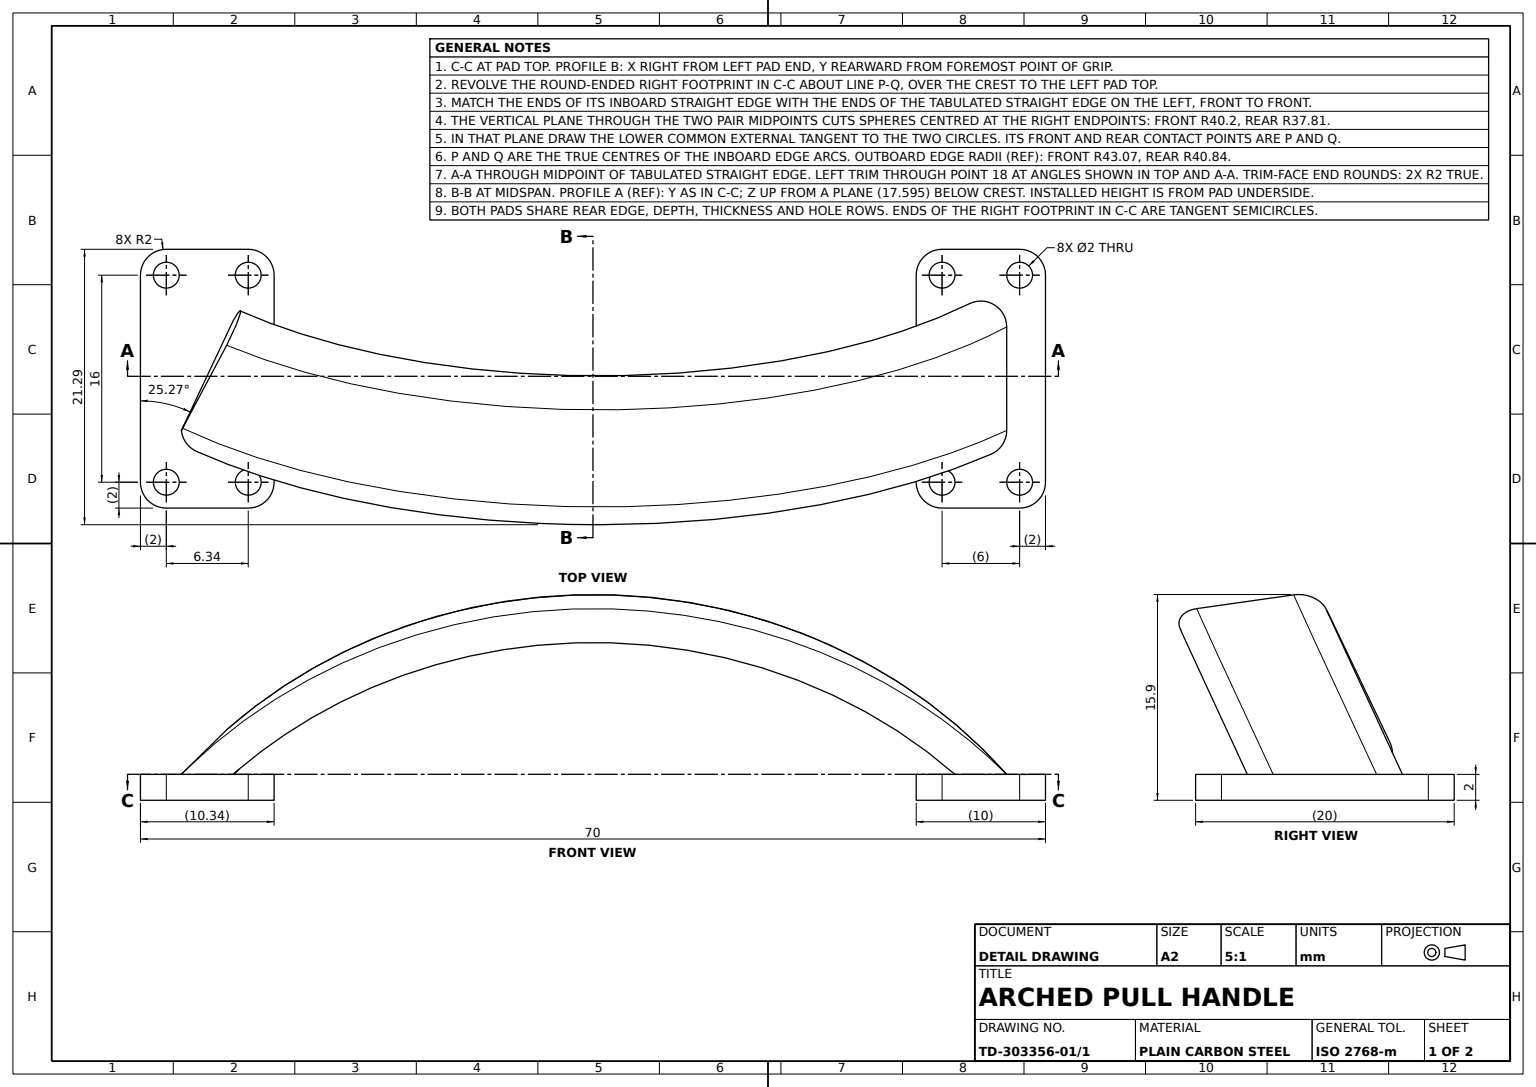
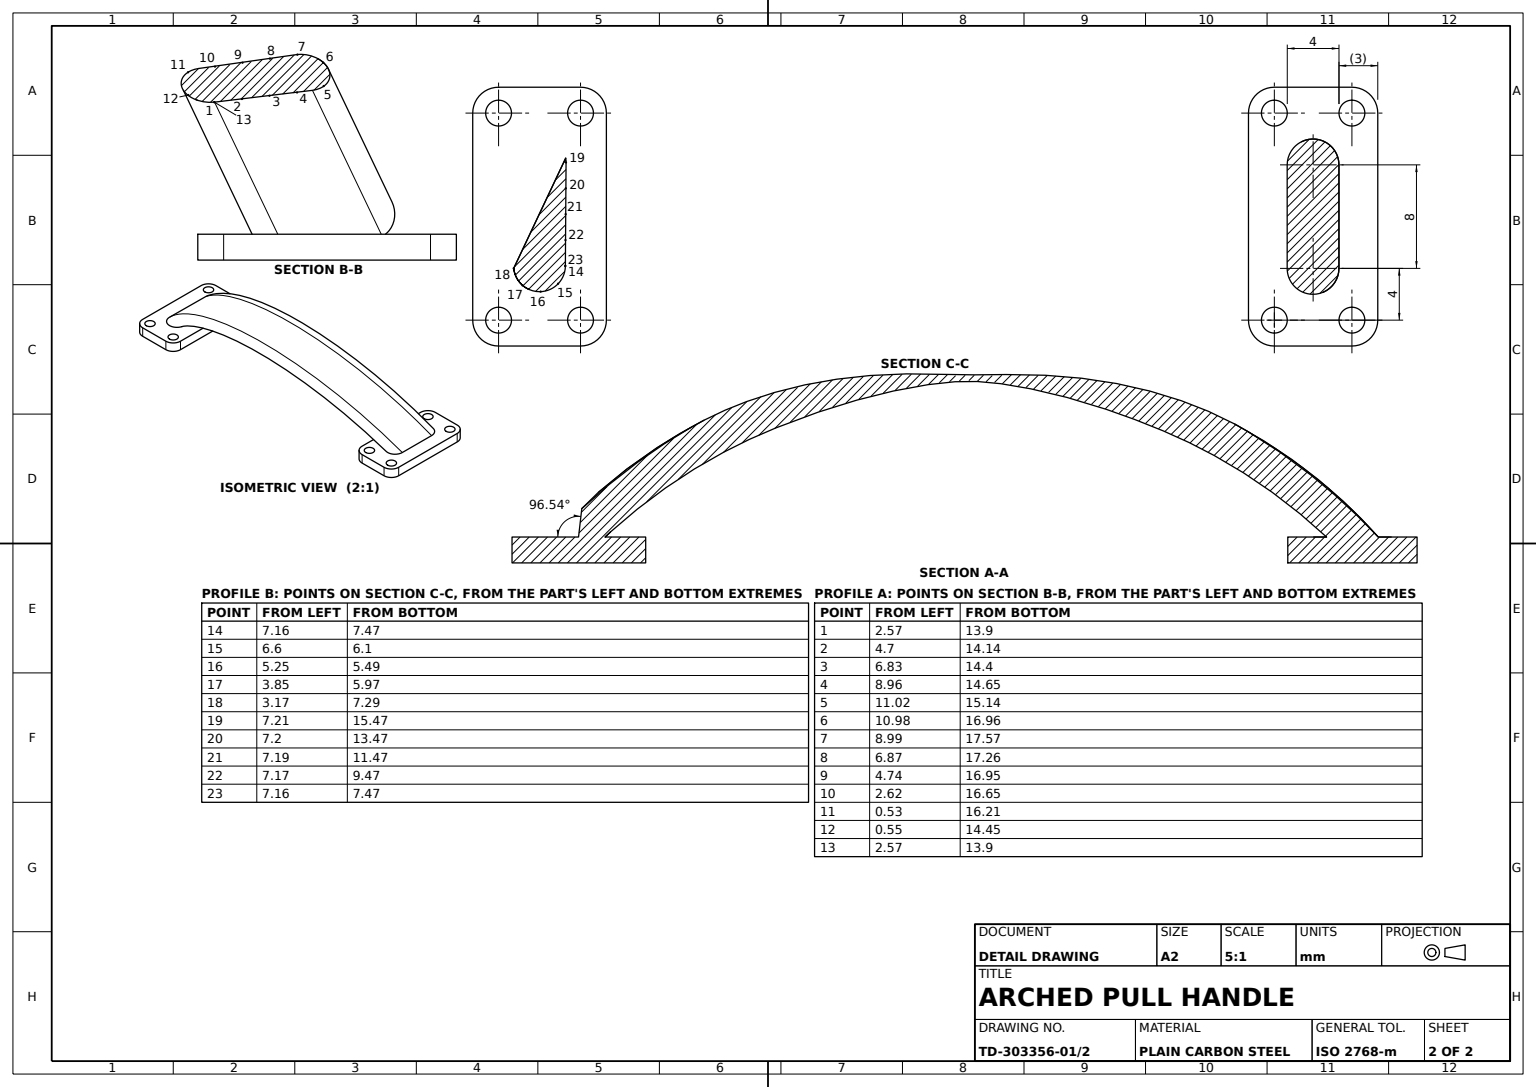
ISO-10303-21;
HEADER;
FILE_DESCRIPTION((''),'2;1');
FILE_NAME('','',(''),(''),'','','');
FILE_SCHEMA(('AUTOMOTIVE_DESIGN'));
ENDSEC;
DATA;
#1=APPLICATION_CONTEXT('');
#2=PRODUCT_CONTEXT('',#1,'mechanical');
#3=PRODUCT('','','',(#2));
#4=PRODUCT_DEFINITION_FORMATION('','',#3);
#5=PRODUCT_DEFINITION_CONTEXT('',#1,'design');
#6=PRODUCT_DEFINITION('','',#4,#5);
#7=PRODUCT_DEFINITION_SHAPE('','',#6);
#8=(LENGTH_UNIT()NAMED_UNIT(*)SI_UNIT(.MILLI.,.METRE.));
#9=(NAMED_UNIT(*)PLANE_ANGLE_UNIT()SI_UNIT($,.RADIAN.));
#10=(NAMED_UNIT(*)SI_UNIT($,.STERADIAN.)SOLID_ANGLE_UNIT());
#11=UNCERTAINTY_MEASURE_WITH_UNIT(LENGTH_MEASURE(1.E-05),#8,'distance_accuracy_value','');
#12=(GEOMETRIC_REPRESENTATION_CONTEXT(3)GLOBAL_UNCERTAINTY_ASSIGNED_CONTEXT((#11))GLOBAL_UNIT_ASSIGNED_CONTEXT((#8,#9,#10))REPRESENTATION_CONTEXT('',''));
#13=CARTESIAN_POINT('',(61.598057,2.,-9.));
#14=VERTEX_POINT('',#13);
#15=CARTESIAN_POINT('',(61.598057,0.,-9.));
#16=VERTEX_POINT('',#15);
#17=CARTESIAN_POINT('',(61.598057,6.,-9.));
#18=DIRECTION('',(0.,-1.,0.));
#19=VECTOR('',#18,1000.);
#20=LINE('',#17,#19);
#21=EDGE_CURVE('',#14,#16,#20,.T.);
#22=ORIENTED_EDGE('',*,*,#21,.T.);
#23=CARTESIAN_POINT('',(61.598057,0.,-7.));
#24=VERTEX_POINT('',#23);
#25=CARTESIAN_POINT('',(61.598057,0.,-8.));
#26=DIRECTION('',(0.,0.,1.));
#27=AXIS2_PLACEMENT_3D('',#25,#18,#26);
#28=CIRCLE('',#27,1.);
#29=EDGE_CURVE('',#16,#24,#28,.T.);
#30=ORIENTED_EDGE('',*,*,#29,.T.);
#31=CARTESIAN_POINT('',(61.598057,2.,-7.));
#32=VERTEX_POINT('',#31);
#33=CARTESIAN_POINT('',(61.598057,6.,-7.));
#34=LINE('',#33,#19);
#35=EDGE_CURVE('',#32,#24,#34,.T.);
#36=ORIENTED_EDGE('',*,*,#35,.F.);
#37=CARTESIAN_POINT('',(61.598057,2.,-8.));
#38=AXIS2_PLACEMENT_3D('',#37,#18,#26);
#39=CIRCLE('',#38,1.);
#40=EDGE_CURVE('',#14,#32,#39,.T.);
#41=ORIENTED_EDGE('',*,*,#40,.F.);
#42=EDGE_LOOP('',(#22,#30,#36,#41));
#43=FACE_OUTER_BOUND('',#42,.T.);
#44=CARTESIAN_POINT('',(61.598057,6.,-8.));
#45=DIRECTION('',(0.,0.,-1.));
#46=AXIS2_PLACEMENT_3D('',#44,#18,#45);
#47=CYLINDRICAL_SURFACE('',#46,1.);
#48=ADVANCED_FACE('',(#43),#47,.F.);
#49=CARTESIAN_POINT('',(61.598057,0.,10.));
#50=VERTEX_POINT('',#49);
#51=CARTESIAN_POINT('',(55.598057,0.,10.));
#52=VERTEX_POINT('',#51);
#53=CARTESIAN_POINT('',(0.,0.,10.));
#54=DIRECTION('',(-1.,0.,0.));
#55=VECTOR('',#54,1000.);
#56=LINE('',#53,#55);
#57=EDGE_CURVE('',#50,#52,#56,.T.);
#58=ORIENTED_EDGE('',*,*,#57,.F.);
#59=CARTESIAN_POINT('',(61.598057,2.,10.));
#60=VERTEX_POINT('',#59);
#61=DIRECTION('',(0.,1.,0.));
#62=VECTOR('',#61,1000.);
#63=LINE('',#49,#62);
#64=EDGE_CURVE('',#50,#60,#63,.T.);
#65=ORIENTED_EDGE('',*,*,#64,.T.);
#66=CARTESIAN_POINT('',(55.598057,2.,10.));
#67=VERTEX_POINT('',#66);
#68=CARTESIAN_POINT('',(0.,2.,10.));
#69=LINE('',#68,#55);
#70=EDGE_CURVE('',#60,#67,#69,.T.);
#71=ORIENTED_EDGE('',*,*,#70,.T.);
#72=LINE('',#51,#62);
#73=EDGE_CURVE('',#52,#67,#72,.T.);
#74=ORIENTED_EDGE('',*,*,#73,.F.);
#75=EDGE_LOOP('',(#58,#65,#71,#74));
#76=FACE_OUTER_BOUND('',#75,.T.);
#77=AXIS2_PLACEMENT_3D('',#53,#45,#54);
#78=PLANE('',#77);
#79=ADVANCED_FACE('',(#76),#78,.F.);
#80=CARTESIAN_POINT('',(1.935999,2.,-7.));
#81=VERTEX_POINT('',#80);
#82=CARTESIAN_POINT('',(1.935999,0.,-7.));
#83=VERTEX_POINT('',#82);
#84=CARTESIAN_POINT('',(1.935999,23.,-7.));
#85=LINE('',#84,#19);
#86=EDGE_CURVE('',#81,#83,#85,.T.);
#87=ORIENTED_EDGE('',*,*,#86,.T.);
#88=CARTESIAN_POINT('',(1.935999,0.,-9.));
#89=VERTEX_POINT('',#88);
#90=CARTESIAN_POINT('',(1.935999,0.,-8.));
#91=AXIS2_PLACEMENT_3D('',#90,#18,#26);
#92=CIRCLE('',#91,1.);
#93=EDGE_CURVE('',#83,#89,#92,.T.);
#94=ORIENTED_EDGE('',*,*,#93,.T.);
#95=CARTESIAN_POINT('',(1.935999,2.,-9.));
#96=VERTEX_POINT('',#95);
#97=CARTESIAN_POINT('',(1.935999,23.,-9.));
#98=LINE('',#97,#19);
#99=EDGE_CURVE('',#96,#89,#98,.T.);
#100=ORIENTED_EDGE('',*,*,#99,.F.);
#101=CARTESIAN_POINT('',(1.935999,2.,-8.));
#102=AXIS2_PLACEMENT_3D('',#101,#18,#26);
#103=CIRCLE('',#102,1.);
#104=EDGE_CURVE('',#81,#96,#103,.T.);
#105=ORIENTED_EDGE('',*,*,#104,.F.);
#106=EDGE_LOOP('',(#87,#94,#100,#105));
#107=FACE_OUTER_BOUND('',#106,.T.);
#108=CARTESIAN_POINT('',(1.935999,23.,-8.));
#109=AXIS2_PLACEMENT_3D('',#108,#18,#45);
#110=CYLINDRICAL_SURFACE('',#109,1.);
#111=ADVANCED_FACE('',(#107),#110,.F.);
#112=CARTESIAN_POINT('',(61.598057,0.,7.));
#113=VERTEX_POINT('',#112);
#114=CARTESIAN_POINT('',(61.598057,0.,9.));
#115=VERTEX_POINT('',#114);
#116=CARTESIAN_POINT('',(61.598057,0.,8.));
#117=AXIS2_PLACEMENT_3D('',#116,#18,#26);
#118=CIRCLE('',#117,1.);
#119=EDGE_CURVE('',#113,#115,#118,.T.);
#120=ORIENTED_EDGE('',*,*,#119,.F.);
#121=EDGE_CURVE('',#115,#113,#118,.T.);
#122=ORIENTED_EDGE('',*,*,#121,.F.);
#123=EDGE_LOOP('',(#120,#122));
#124=FACE_BOUND('',#123,.T.);
#125=CARTESIAN_POINT('',(55.598057,0.,-9.));
#126=VERTEX_POINT('',#125);
#127=CARTESIAN_POINT('',(55.598057,0.,-7.));
#128=VERTEX_POINT('',#127);
#129=CARTESIAN_POINT('',(55.598057,0.,-8.));
#130=AXIS2_PLACEMENT_3D('',#129,#18,#26);
#131=CIRCLE('',#130,1.);
#132=EDGE_CURVE('',#126,#128,#131,.T.);
#133=ORIENTED_EDGE('',*,*,#132,.F.);
#134=EDGE_CURVE('',#128,#126,#131,.T.);
#135=ORIENTED_EDGE('',*,*,#134,.F.);
#136=EDGE_LOOP('',(#133,#135));
#137=FACE_BOUND('',#136,.T.);
#138=CARTESIAN_POINT('',(63.598057,0.,8.));
#139=VERTEX_POINT('',#138);
#140=CIRCLE('',#117,2.);
#141=EDGE_CURVE('',#139,#50,#140,.T.);
#142=ORIENTED_EDGE('',*,*,#141,.T.);
#143=ORIENTED_EDGE('',*,*,#57,.T.);
#144=CARTESIAN_POINT('',(53.598057,0.,8.));
#145=VERTEX_POINT('',#144);
#146=CARTESIAN_POINT('',(55.598057,0.,8.));
#147=AXIS2_PLACEMENT_3D('',#146,#18,#26);
#148=CIRCLE('',#147,2.);
#149=EDGE_CURVE('',#52,#145,#148,.T.);
#150=ORIENTED_EDGE('',*,*,#149,.T.);
#151=CARTESIAN_POINT('',(53.598057,0.,-8.));
#152=VERTEX_POINT('',#151);
#153=CARTESIAN_POINT('',(53.598057,0.,0.));
#154=VECTOR('',#26,1000.);
#155=LINE('',#153,#154);
#156=EDGE_CURVE('',#152,#145,#155,.T.);
#157=ORIENTED_EDGE('',*,*,#156,.F.);
#158=CARTESIAN_POINT('',(55.598057,0.,-10.));
#159=VERTEX_POINT('',#158);
#160=AXIS2_PLACEMENT_3D('',#129,#61,#26);
#161=CIRCLE('',#160,2.);
#162=EDGE_CURVE('',#159,#152,#161,.T.);
#163=ORIENTED_EDGE('',*,*,#162,.F.);
#164=CARTESIAN_POINT('',(61.598057,0.,-10.));
#165=VERTEX_POINT('',#164);
#166=CARTESIAN_POINT('',(0.,0.,-10.));
#167=LINE('',#166,#55);
#168=EDGE_CURVE('',#165,#159,#167,.T.);
#169=ORIENTED_EDGE('',*,*,#168,.F.);
#170=CARTESIAN_POINT('',(63.598057,0.,-8.));
#171=VERTEX_POINT('',#170);
#172=CIRCLE('',#27,2.);
#173=EDGE_CURVE('',#165,#171,#172,.T.);
#174=ORIENTED_EDGE('',*,*,#173,.T.);
#175=CARTESIAN_POINT('',(63.598057,0.,0.));
#176=LINE('',#175,#154);
#177=EDGE_CURVE('',#171,#139,#176,.T.);
#178=ORIENTED_EDGE('',*,*,#177,.T.);
#179=EDGE_LOOP('',(#142,#143,#150,#157,#163,#169,#174,#178));
#180=FACE_OUTER_BOUND('',#179,.T.);
#181=EDGE_CURVE('',#24,#16,#28,.T.);
#182=ORIENTED_EDGE('',*,*,#181,.F.);
#183=ORIENTED_EDGE('',*,*,#29,.F.);
#184=EDGE_LOOP('',(#182,#183));
#185=FACE_BOUND('',#184,.T.);
#186=CARTESIAN_POINT('',(55.598057,0.,7.));
#187=VERTEX_POINT('',#186);
#188=CARTESIAN_POINT('',(55.598057,0.,9.));
#189=VERTEX_POINT('',#188);
#190=CIRCLE('',#147,1.);
#191=EDGE_CURVE('',#187,#189,#190,.T.);
#192=ORIENTED_EDGE('',*,*,#191,.F.);
#193=EDGE_CURVE('',#189,#187,#190,.T.);
#194=ORIENTED_EDGE('',*,*,#193,.F.);
#195=EDGE_LOOP('',(#192,#194));
#196=FACE_BOUND('',#195,.T.);
#197=CARTESIAN_POINT('',(0.,0.,0.));
#198=AXIS2_PLACEMENT_3D('',#197,#61,#26);
#199=PLANE('',#198);
#200=ADVANCED_FACE('',(#124,#137,#180,#185,#196),#199,.F.);
#201=CARTESIAN_POINT('',(-4.401943,0.,-10.));
#202=VERTEX_POINT('',#201);
#203=CARTESIAN_POINT('',(-6.401943,0.,-8.));
#204=VERTEX_POINT('',#203);
#205=CARTESIAN_POINT('',(-4.401943,0.,-8.));
#206=AXIS2_PLACEMENT_3D('',#205,#61,#26);
#207=CIRCLE('',#206,2.);
#208=EDGE_CURVE('',#202,#204,#207,.T.);
#209=ORIENTED_EDGE('',*,*,#208,.F.);
#210=CARTESIAN_POINT('',(1.935999,0.,-10.));
#211=VERTEX_POINT('',#210);
#212=LINE('',#201,#55);
#213=EDGE_CURVE('',#211,#202,#212,.T.);
#214=ORIENTED_EDGE('',*,*,#213,.F.);
#215=CARTESIAN_POINT('',(3.935999,0.,-8.));
#216=VERTEX_POINT('',#215);
#217=AXIS2_PLACEMENT_3D('',#90,#61,#26);
#218=CIRCLE('',#217,2.);
#219=EDGE_CURVE('',#216,#211,#218,.T.);
#220=ORIENTED_EDGE('',*,*,#219,.F.);
#221=CARTESIAN_POINT('',(3.935999,0.,8.));
#222=VERTEX_POINT('',#221);
#223=VECTOR('',#45,1000.);
#224=LINE('',#215,#223);
#225=EDGE_CURVE('',#222,#216,#224,.T.);
#226=ORIENTED_EDGE('',*,*,#225,.F.);
#227=CARTESIAN_POINT('',(1.935999,0.,10.));
#228=VERTEX_POINT('',#227);
#229=CARTESIAN_POINT('',(1.935999,0.,8.));
#230=AXIS2_PLACEMENT_3D('',#229,#61,#26);
#231=CIRCLE('',#230,2.);
#232=EDGE_CURVE('',#228,#222,#231,.T.);
#233=ORIENTED_EDGE('',*,*,#232,.F.);
#234=CARTESIAN_POINT('',(-4.401943,0.,10.));
#235=VERTEX_POINT('',#234);
#236=DIRECTION('',(1.,0.,0.));
#237=VECTOR('',#236,1000.);
#238=LINE('',#234,#237);
#239=EDGE_CURVE('',#235,#228,#238,.T.);
#240=ORIENTED_EDGE('',*,*,#239,.F.);
#241=CARTESIAN_POINT('',(-6.401943,0.,8.));
#242=VERTEX_POINT('',#241);
#243=CARTESIAN_POINT('',(-4.401943,0.,8.));
#244=AXIS2_PLACEMENT_3D('',#243,#61,#26);
#245=CIRCLE('',#244,2.);
#246=EDGE_CURVE('',#242,#235,#245,.T.);
#247=ORIENTED_EDGE('',*,*,#246,.F.);
#248=LINE('',#203,#154);
#249=EDGE_CURVE('',#204,#242,#248,.T.);
#250=ORIENTED_EDGE('',*,*,#249,.F.);
#251=EDGE_LOOP('',(#209,#214,#220,#226,#233,#240,#247,#250));
#252=FACE_OUTER_BOUND('',#251,.T.);
#253=CARTESIAN_POINT('',(-4.401943,0.,7.));
#254=VERTEX_POINT('',#253);
#255=CARTESIAN_POINT('',(-4.401943,0.,9.));
#256=VERTEX_POINT('',#255);
#257=AXIS2_PLACEMENT_3D('',#243,#18,#26);
#258=CIRCLE('',#257,1.);
#259=EDGE_CURVE('',#254,#256,#258,.T.);
#260=ORIENTED_EDGE('',*,*,#259,.F.);
#261=EDGE_CURVE('',#256,#254,#258,.T.);
#262=ORIENTED_EDGE('',*,*,#261,.F.);
#263=EDGE_LOOP('',(#260,#262));
#264=FACE_BOUND('',#263,.T.);
#265=CARTESIAN_POINT('',(1.935999,0.,9.));
#266=VERTEX_POINT('',#265);
#267=CARTESIAN_POINT('',(1.935999,0.,7.));
#268=VERTEX_POINT('',#267);
#269=AXIS2_PLACEMENT_3D('',#229,#18,#26);
#270=CIRCLE('',#269,1.);
#271=EDGE_CURVE('',#266,#268,#270,.T.);
#272=ORIENTED_EDGE('',*,*,#271,.F.);
#273=EDGE_CURVE('',#268,#266,#270,.T.);
#274=ORIENTED_EDGE('',*,*,#273,.F.);
#275=EDGE_LOOP('',(#272,#274));
#276=FACE_BOUND('',#275,.T.);
#277=CARTESIAN_POINT('',(-4.401943,0.,-9.));
#278=VERTEX_POINT('',#277);
#279=CARTESIAN_POINT('',(-4.401943,0.,-7.));
#280=VERTEX_POINT('',#279);
#281=AXIS2_PLACEMENT_3D('',#205,#18,#26);
#282=CIRCLE('',#281,1.);
#283=EDGE_CURVE('',#278,#280,#282,.T.);
#284=ORIENTED_EDGE('',*,*,#283,.F.);
#285=EDGE_CURVE('',#280,#278,#282,.T.);
#286=ORIENTED_EDGE('',*,*,#285,.F.);
#287=EDGE_LOOP('',(#284,#286));
#288=FACE_BOUND('',#287,.T.);
#289=ORIENTED_EDGE('',*,*,#93,.F.);
#290=EDGE_CURVE('',#89,#83,#92,.T.);
#291=ORIENTED_EDGE('',*,*,#290,.F.);
#292=EDGE_LOOP('',(#289,#291));
#293=FACE_BOUND('',#292,.T.);
#294=PLANE('',#206);
#295=ADVANCED_FACE('',(#252,#264,#276,#288,#293),#294,.F.);
#296=CARTESIAN_POINT('',(55.598057,2.,-7.));
#297=VERTEX_POINT('',#296);
#298=CARTESIAN_POINT('',(55.598057,2.,-9.));
#299=VERTEX_POINT('',#298);
#300=CARTESIAN_POINT('',(55.598057,2.,-8.));
#301=AXIS2_PLACEMENT_3D('',#300,#18,#26);
#302=CIRCLE('',#301,1.);
#303=EDGE_CURVE('',#297,#299,#302,.T.);
#304=ORIENTED_EDGE('',*,*,#303,.F.);
#305=CARTESIAN_POINT('',(55.598057,6.,-7.));
#306=LINE('',#305,#19);
#307=EDGE_CURVE('',#297,#128,#306,.T.);
#308=ORIENTED_EDGE('',*,*,#307,.T.);
#309=ORIENTED_EDGE('',*,*,#134,.T.);
#310=CARTESIAN_POINT('',(55.598057,6.,-9.));
#311=LINE('',#310,#19);
#312=EDGE_CURVE('',#299,#126,#311,.T.);
#313=ORIENTED_EDGE('',*,*,#312,.F.);
#314=EDGE_LOOP('',(#304,#308,#309,#313));
#315=FACE_OUTER_BOUND('',#314,.T.);
#316=CARTESIAN_POINT('',(55.598057,6.,-8.));
#317=AXIS2_PLACEMENT_3D('',#316,#18,#45);
#318=CYLINDRICAL_SURFACE('',#317,1.);
#319=ADVANCED_FACE('',(#315),#318,.F.);
#320=ORIENTED_EDGE('',*,*,#285,.T.);
#321=CARTESIAN_POINT('',(-4.401943,2.,-9.));
#322=VERTEX_POINT('',#321);
#323=CARTESIAN_POINT('',(-4.401943,17.,-9.));
#324=LINE('',#323,#19);
#325=EDGE_CURVE('',#322,#278,#324,.T.);
#326=ORIENTED_EDGE('',*,*,#325,.F.);
#327=CARTESIAN_POINT('',(-4.401943,2.,-7.));
#328=VERTEX_POINT('',#327);
#329=CARTESIAN_POINT('',(-4.401943,2.,-8.));
#330=AXIS2_PLACEMENT_3D('',#329,#18,#26);
#331=CIRCLE('',#330,1.);
#332=EDGE_CURVE('',#328,#322,#331,.T.);
#333=ORIENTED_EDGE('',*,*,#332,.F.);
#334=CARTESIAN_POINT('',(-4.401943,17.,-7.));
#335=LINE('',#334,#19);
#336=EDGE_CURVE('',#328,#280,#335,.T.);
#337=ORIENTED_EDGE('',*,*,#336,.T.);
#338=EDGE_LOOP('',(#320,#326,#333,#337));
#339=FACE_OUTER_BOUND('',#338,.T.);
#340=CARTESIAN_POINT('',(-4.401943,17.,-8.));
#341=AXIS2_PLACEMENT_3D('',#340,#18,#45);
#342=CYLINDRICAL_SURFACE('',#341,1.);
#343=ADVANCED_FACE('',(#339),#342,.F.);
#344=CARTESIAN_POINT('',(0.786093,2.,-4.514668));
#345=VERTEX_POINT('',#344);
#346=CARTESIAN_POINT('',(-3.232972,2.,4.));
#347=VERTEX_POINT('',#346);
#348=CARTESIAN_POINT('',(1.186193,2.,-5.362307));
#349=DIRECTION('',(-0.426854324,0.,0.9043204));
#350=VECTOR('',#349,1000.);
#351=LINE('',#348,#350);
#352=EDGE_CURVE('',#345,#347,#351,.T.);
#353=ORIENTED_EDGE('',*,*,#352,.T.);
#354=CARTESIAN_POINT('',(-3.142334,2.100495,3.832389));
#355=VERTEX_POINT('',#354);
#356=CARTESIAN_POINT('',(-2.95236,0.295815,2.99153));
#357=DIRECTION('',(-0.899497793,0.103137123,-0.424577973));
#358=DIRECTION('',(-0.426475367,-0.418504621,0.80185575));
#359=AXIS2_PLACEMENT_3D('',#356,#357,#358);
#360=CIRCLE('',#359,2.);
#361=EDGE_CURVE('',#347,#355,#360,.T.);
#362=ORIENTED_EDGE('',*,*,#361,.T.);
#363=CARTESIAN_POINT('',(0.269469,5.448532,-2.582457));
#364=VERTEX_POINT('',#363);
#365=DIRECTION('',(0.426475367,0.418504621,-0.80185575));
#366=VECTOR('',#365,1000.);
#367=LINE('',#363,#366);
#368=EDGE_CURVE('',#355,#364,#367,.T.);
#369=ORIENTED_EDGE('',*,*,#368,.T.);
#370=CARTESIAN_POINT('',(0.459442,3.643852,-3.423316));
#371=AXIS2_PLACEMENT_3D('',#370,#357,#358);
#372=CIRCLE('',#371,2.);
#373=EDGE_CURVE('',#364,#345,#372,.T.);
#374=ORIENTED_EDGE('',*,*,#373,.T.);
#375=EDGE_LOOP('',(#353,#362,#369,#374));
#376=FACE_OUTER_BOUND('',#375,.T.);
#377=PLANE('',#371);
#378=ADVANCED_FACE('',(#376),#377,.T.);
#379=ORIENTED_EDGE('',*,*,#35,.T.);
#380=ORIENTED_EDGE('',*,*,#181,.T.);
#381=ORIENTED_EDGE('',*,*,#21,.F.);
#382=EDGE_CURVE('',#32,#14,#39,.T.);
#383=ORIENTED_EDGE('',*,*,#382,.F.);
#384=EDGE_LOOP('',(#379,#380,#381,#383));
#385=FACE_OUTER_BOUND('',#384,.T.);
#386=ADVANCED_FACE('',(#385),#47,.F.);
#387=EDGE_CURVE('',#322,#328,#331,.T.);
#388=ORIENTED_EDGE('',*,*,#387,.F.);
#389=ORIENTED_EDGE('',*,*,#325,.T.);
#390=ORIENTED_EDGE('',*,*,#283,.T.);
#391=ORIENTED_EDGE('',*,*,#336,.F.);
#392=EDGE_LOOP('',(#388,#389,#390,#391));
#393=FACE_OUTER_BOUND('',#392,.T.);
#394=ADVANCED_FACE('',(#393),#342,.F.);
#395=CARTESIAN_POINT('',(63.598057,2.,-8.));
#396=VERTEX_POINT('',#395);
#397=LINE('',#170,#62);
#398=EDGE_CURVE('',#171,#396,#397,.T.);
#399=ORIENTED_EDGE('',*,*,#398,.F.);
#400=ORIENTED_EDGE('',*,*,#173,.F.);
#401=CARTESIAN_POINT('',(61.598057,2.,-10.));
#402=VERTEX_POINT('',#401);
#403=LINE('',#164,#62);
#404=EDGE_CURVE('',#165,#402,#403,.T.);
#405=ORIENTED_EDGE('',*,*,#404,.T.);
#406=CIRCLE('',#38,2.);
#407=EDGE_CURVE('',#402,#396,#406,.T.);
#408=ORIENTED_EDGE('',*,*,#407,.T.);
#409=EDGE_LOOP('',(#399,#400,#405,#408));
#410=FACE_OUTER_BOUND('',#409,.T.);
#411=AXIS2_PLACEMENT_3D('',#25,#61,#26);
#412=CYLINDRICAL_SURFACE('',#411,2.);
#413=ADVANCED_FACE('',(#410),#412,.T.);
#414=ORIENTED_EDGE('',*,*,#239,.T.);
#415=CARTESIAN_POINT('',(1.935999,2.,10.));
#416=VERTEX_POINT('',#415);
#417=LINE('',#415,#19);
#418=EDGE_CURVE('',#416,#228,#417,.T.);
#419=ORIENTED_EDGE('',*,*,#418,.F.);
#420=CARTESIAN_POINT('',(-4.401943,2.,10.));
#421=VERTEX_POINT('',#420);
#422=LINE('',#420,#237);
#423=EDGE_CURVE('',#421,#416,#422,.T.);
#424=ORIENTED_EDGE('',*,*,#423,.F.);
#425=LINE('',#420,#19);
#426=EDGE_CURVE('',#421,#235,#425,.T.);
#427=ORIENTED_EDGE('',*,*,#426,.T.);
#428=EDGE_LOOP('',(#414,#419,#424,#427));
#429=FACE_OUTER_BOUND('',#428,.T.);
#430=AXIS2_PLACEMENT_3D('',#420,#45,#54);
#431=PLANE('',#430);
#432=ADVANCED_FACE('',(#429),#431,.F.);
#433=CARTESIAN_POINT('',(55.598057,2.,9.));
#434=VERTEX_POINT('',#433);
#435=CARTESIAN_POINT('',(55.598057,6.,9.));
#436=LINE('',#435,#19);
#437=EDGE_CURVE('',#434,#189,#436,.T.);
#438=ORIENTED_EDGE('',*,*,#437,.T.);
#439=ORIENTED_EDGE('',*,*,#193,.T.);
#440=CARTESIAN_POINT('',(55.598057,2.,7.));
#441=VERTEX_POINT('',#440);
#442=CARTESIAN_POINT('',(55.598057,6.,7.));
#443=LINE('',#442,#19);
#444=EDGE_CURVE('',#441,#187,#443,.T.);
#445=ORIENTED_EDGE('',*,*,#444,.F.);
#446=CARTESIAN_POINT('',(55.598057,2.,8.));
#447=AXIS2_PLACEMENT_3D('',#446,#18,#26);
#448=CIRCLE('',#447,1.);
#449=EDGE_CURVE('',#434,#441,#448,.T.);
#450=ORIENTED_EDGE('',*,*,#449,.F.);
#451=EDGE_LOOP('',(#438,#439,#445,#450));
#452=FACE_OUTER_BOUND('',#451,.T.);
#453=CARTESIAN_POINT('',(55.598057,6.,8.));
#454=AXIS2_PLACEMENT_3D('',#453,#18,#45);
#455=CYLINDRICAL_SURFACE('',#454,1.);
#456=ADVANCED_FACE('',(#452),#455,.F.);
#457=CARTESIAN_POINT('',(53.598057,2.,-8.));
#458=VERTEX_POINT('',#457);
#459=LINE('',#151,#62);
#460=EDGE_CURVE('',#152,#458,#459,.T.);
#461=ORIENTED_EDGE('',*,*,#460,.T.);
#462=CARTESIAN_POINT('',(55.598057,2.,-10.));
#463=VERTEX_POINT('',#462);
#464=AXIS2_PLACEMENT_3D('',#300,#61,#26);
#465=CIRCLE('',#464,2.);
#466=EDGE_CURVE('',#463,#458,#465,.T.);
#467=ORIENTED_EDGE('',*,*,#466,.F.);
#468=LINE('',#158,#62);
#469=EDGE_CURVE('',#159,#463,#468,.T.);
#470=ORIENTED_EDGE('',*,*,#469,.F.);
#471=ORIENTED_EDGE('',*,*,#162,.T.);
#472=EDGE_LOOP('',(#461,#467,#470,#471));
#473=FACE_OUTER_BOUND('',#472,.T.);
#474=CYLINDRICAL_SURFACE('',#160,2.);
#475=ADVANCED_FACE('',(#473),#474,.T.);
#476=CARTESIAN_POINT('',(61.598057,2.,9.));
#477=VERTEX_POINT('',#476);
#478=CARTESIAN_POINT('',(61.598057,2.,7.));
#479=VERTEX_POINT('',#478);
#480=CARTESIAN_POINT('',(61.598057,2.,8.));
#481=AXIS2_PLACEMENT_3D('',#480,#18,#26);
#482=CIRCLE('',#481,1.);
#483=EDGE_CURVE('',#477,#479,#482,.T.);
#484=ORIENTED_EDGE('',*,*,#483,.F.);
#485=CARTESIAN_POINT('',(61.598057,6.,9.));
#486=LINE('',#485,#19);
#487=EDGE_CURVE('',#477,#115,#486,.T.);
#488=ORIENTED_EDGE('',*,*,#487,.T.);
#489=ORIENTED_EDGE('',*,*,#121,.T.);
#490=CARTESIAN_POINT('',(61.598057,6.,7.));
#491=LINE('',#490,#19);
#492=EDGE_CURVE('',#479,#113,#491,.T.);
#493=ORIENTED_EDGE('',*,*,#492,.F.);
#494=EDGE_LOOP('',(#484,#488,#489,#493));
#495=FACE_OUTER_BOUND('',#494,.T.);
#496=CARTESIAN_POINT('',(61.598057,6.,8.));
#497=AXIS2_PLACEMENT_3D('',#496,#18,#45);
#498=CYLINDRICAL_SURFACE('',#497,1.);
#499=ADVANCED_FACE('',(#495),#498,.F.);
#500=CARTESIAN_POINT('',(-6.401943,2.,-8.));
#501=VERTEX_POINT('',#500);
#502=LINE('',#500,#19);
#503=EDGE_CURVE('',#501,#204,#502,.T.);
#504=ORIENTED_EDGE('',*,*,#503,.T.);
#505=ORIENTED_EDGE('',*,*,#249,.T.);
#506=CARTESIAN_POINT('',(-6.401943,2.,8.));
#507=VERTEX_POINT('',#506);
#508=LINE('',#506,#19);
#509=EDGE_CURVE('',#507,#242,#508,.T.);
#510=ORIENTED_EDGE('',*,*,#509,.F.);
#511=LINE('',#500,#154);
#512=EDGE_CURVE('',#501,#507,#511,.T.);
#513=ORIENTED_EDGE('',*,*,#512,.F.);
#514=EDGE_LOOP('',(#504,#505,#510,#513));
#515=FACE_OUTER_BOUND('',#514,.T.);
#516=AXIS2_PLACEMENT_3D('',#500,#236,#45);
#517=PLANE('',#516);
#518=ADVANCED_FACE('',(#515),#517,.F.);
#519=CARTESIAN_POINT('',(-4.401943,2.,9.));
#520=VERTEX_POINT('',#519);
#521=CARTESIAN_POINT('',(-4.401943,2.,7.));
#522=VERTEX_POINT('',#521);
#523=CARTESIAN_POINT('',(-4.401943,2.,8.));
#524=AXIS2_PLACEMENT_3D('',#523,#18,#26);
#525=CIRCLE('',#524,1.);
#526=EDGE_CURVE('',#520,#522,#525,.T.);
#527=ORIENTED_EDGE('',*,*,#526,.F.);
#528=CARTESIAN_POINT('',(-4.401943,25.,9.));
#529=LINE('',#528,#19);
#530=EDGE_CURVE('',#520,#256,#529,.T.);
#531=ORIENTED_EDGE('',*,*,#530,.T.);
#532=ORIENTED_EDGE('',*,*,#261,.T.);
#533=CARTESIAN_POINT('',(-4.401943,25.,7.));
#534=LINE('',#533,#19);
#535=EDGE_CURVE('',#522,#254,#534,.T.);
#536=ORIENTED_EDGE('',*,*,#535,.F.);
#537=EDGE_LOOP('',(#527,#531,#532,#536));
#538=FACE_OUTER_BOUND('',#537,.T.);
#539=CARTESIAN_POINT('',(-4.401943,25.,8.));
#540=AXIS2_PLACEMENT_3D('',#539,#18,#45);
#541=CYLINDRICAL_SURFACE('',#540,1.);
#542=ADVANCED_FACE('',(#538),#541,.F.);
#543=CARTESIAN_POINT('',(53.598057,2.,8.));
#544=VERTEX_POINT('',#543);
#545=CARTESIAN_POINT('',(53.598057,2.,0.));
#546=LINE('',#545,#154);
#547=EDGE_CURVE('',#458,#544,#546,.T.);
#548=ORIENTED_EDGE('',*,*,#547,.F.);
#549=ORIENTED_EDGE('',*,*,#460,.F.);
#550=ORIENTED_EDGE('',*,*,#156,.T.);
#551=LINE('',#144,#62);
#552=EDGE_CURVE('',#145,#544,#551,.T.);
#553=ORIENTED_EDGE('',*,*,#552,.T.);
#554=EDGE_LOOP('',(#548,#549,#550,#553));
#555=FACE_OUTER_BOUND('',#554,.T.);
#556=AXIS2_PLACEMENT_3D('',#153,#54,#26);
#557=PLANE('',#556);
#558=ADVANCED_FACE('',(#555),#557,.T.);
#559=ORIENTED_EDGE('',*,*,#509,.T.);
#560=ORIENTED_EDGE('',*,*,#246,.T.);
#561=ORIENTED_EDGE('',*,*,#426,.F.);
#562=AXIS2_PLACEMENT_3D('',#523,#61,#26);
#563=CIRCLE('',#562,2.);
#564=EDGE_CURVE('',#507,#421,#563,.T.);
#565=ORIENTED_EDGE('',*,*,#564,.F.);
#566=EDGE_LOOP('',(#559,#560,#561,#565));
#567=FACE_OUTER_BOUND('',#566,.T.);
#568=AXIS2_PLACEMENT_3D('',#523,#18,#45);
#569=CYLINDRICAL_SURFACE('',#568,2.);
#570=ADVANCED_FACE('',(#567),#569,.T.);
#571=ORIENTED_EDGE('',*,*,#373,.F.);
#572=CARTESIAN_POINT('',(60.598057,2.,-4.));
#573=VERTEX_POINT('',#572);
#574=CARTESIAN_POINT('',(28.741015,-21.091715,-14.961014));
#575=DIRECTION('',(0.003050471,0.425376132,-0.905011514));
#576=DIRECTION('',(-0.697078179,0.649793546,0.303068242));
#577=AXIS2_PLACEMENT_3D('',#574,#575,#576);
#578=CIRCLE('',#577,40.844122);
#579=EDGE_CURVE('',#364,#573,#578,.T.);
#580=ORIENTED_EDGE('',*,*,#579,.T.);
#581=CARTESIAN_POINT('',(56.598057,2.,-4.));
#582=VERTEX_POINT('',#581);
#583=CARTESIAN_POINT('',(58.598057,2.,-4.));
#584=AXIS2_PLACEMENT_3D('',#583,#61,#26);
#585=CIRCLE('',#584,2.);
#586=EDGE_CURVE('',#573,#582,#585,.T.);
#587=ORIENTED_EDGE('',*,*,#586,.T.);
#588=CARTESIAN_POINT('',(0.810715,2.,-4.188039));
#589=VERTEX_POINT('',#588);
#590=CARTESIAN_POINT('',(28.740978,-21.096906,-14.949971));
#591=DIRECTION('',(-0.743021113,0.606658721,0.282639029));
#592=AXIS2_PLACEMENT_3D('',#590,#575,#591);
#593=CIRCLE('',#592,37.807219);
#594=EDGE_CURVE('',#589,#582,#593,.T.);
#595=ORIENTED_EDGE('',*,*,#594,.F.);
#596=CARTESIAN_POINT('',(0.803246,2.,-4.406466));
#597=CARTESIAN_POINT('',(0.811454,2.,-4.29759));
#598=B_SPLINE_CURVE_WITH_KNOTS('',3,(#344,#596,#597,#588),.UNSPECIFIED.,.F.,.F.,(4,4),(0.,0.000327555),.UNSPECIFIED.);
#599=EDGE_CURVE('',#345,#589,#598,.T.);
#600=ORIENTED_EDGE('',*,*,#599,.F.);
#601=EDGE_LOOP('',(#571,#580,#587,#595,#600));
#602=FACE_OUTER_BOUND('',#601,.T.);
#603=CARTESIAN_POINT('',(18.747381,21.683046,5.110419));
#604=CARTESIAN_POINT('',(44.469858,20.212686,4.506017));
#605=CARTESIAN_POINT('',(1.97537,7.12255,-5.78988));
#606=CARTESIAN_POINT('',(20.548336,22.389104,1.448352));
#607=CARTESIAN_POINT('',(45.543462,20.204987,0.506017));
#608=CARTESIAN_POINT('',(60.598057,2.,-8.));
#609=CARTESIAN_POINT('',(2.355317,3.513192,-7.471598));
#610=CARTESIAN_POINT('',(18.415827,18.566018,-0.342291));
#611=CARTESIAN_POINT('',(41.543462,17.920834,-0.567587));
#612=CARTESIAN_POINT('',(56.598057,2.,-8.));
#613=CARTESIAN_POINT('',(0.649416,1.839173,-4.264175));
#614=CARTESIAN_POINT('',(16.614872,17.859961,3.319776));
#615=CARTESIAN_POINT('',(40.469858,17.928533,3.432413));
#616=(BOUNDED_SURFACE()B_SPLINE_SURFACE(3,3,((#363,#603,#604,#572),(#605,#606,#607,#608),(#609,#610,#611,#612),(#613,#614,#615,#581)),.UNSPECIFIED.,.F.,.F.,.T.)B_SPLINE_SURFACE_WITH_KNOTS((4,4),(4,4),(0.,1.),(0.,1.),.UNSPECIFIED.)GEOMETRIC_REPRESENTATION_ITEM()RATIONAL_B_SPLINE_SURFACE(((1.,0.781788227,0.781788227,1.),(0.333333333,0.260596076,0.260596076,0.333333333),(0.333333333,0.260596076,0.260596076,0.333333333),(1.,0.781788227,0.781788227,1.)))REPRESENTATION_ITEM('')SURFACE());
#617=ADVANCED_FACE('',(#602),#616,.F.);
#618=CARTESIAN_POINT('',(56.598057,2.,4.));
#619=VERTEX_POINT('',#618);
#620=LINE('',#581,#154);
#621=EDGE_CURVE('',#582,#619,#620,.T.);
#622=ORIENTED_EDGE('',*,*,#621,.T.);
#623=CARTESIAN_POINT('',(0.756785,2.,3.811779));
#624=VERTEX_POINT('',#623);
#625=CARTESIAN_POINT('',(28.718892,-24.176668,-8.397604));
#626=DIRECTION('',(-0.783085772,0.563853683,0.262384637));
#627=AXIS2_PLACEMENT_3D('',#625,#575,#626);
#628=CIRCLE('',#627,40.201572);
#629=EDGE_CURVE('',#624,#619,#628,.T.);
#630=ORIENTED_EDGE('',*,*,#629,.F.);
#631=CARTESIAN_POINT('',(0.806062,2.,-3.497792));
#632=CARTESIAN_POINT('',(0.801409,2.,-2.807544));
#633=CARTESIAN_POINT('',(0.796755,2.,-2.117296));
#634=CARTESIAN_POINT('',(0.792102,2.,-1.427049));
#635=CARTESIAN_POINT('',(0.787449,2.,-0.736801));
#636=CARTESIAN_POINT('',(0.782796,2.,-0.046553));
#637=CARTESIAN_POINT('',(0.774126,2.,1.239557));
#638=CARTESIAN_POINT('',(0.765456,2.,2.525668));
#639=B_SPLINE_CURVE_WITH_KNOTS('',3,(#588,#631,#632,#633,#634,#635,#636,#637,#638,#623),.UNSPECIFIED.,.F.,.F.,(4,3,3,4),(0.,0.00207079,0.00414158,0.008),.UNSPECIFIED.);
#640=EDGE_CURVE('',#589,#624,#639,.T.);
#641=ORIENTED_EDGE('',*,*,#640,.F.);
#642=ORIENTED_EDGE('',*,*,#594,.T.);
#643=EDGE_LOOP('',(#622,#630,#641,#642));
#644=FACE_OUTER_BOUND('',#643,.T.);
#645=CARTESIAN_POINT('',(-2.762387,-1.508864,2.150671));
#646=CARTESIAN_POINT('',(13.012964,16.447847,10.643909));
#647=CARTESIAN_POINT('',(38.32265,17.943931,11.432413));
#648=(BOUNDED_SURFACE()B_SPLINE_SURFACE(1,3,((#613,#614,#615,#581),(#645,#646,#647,#618)),.UNSPECIFIED.,.F.,.F.,.T.)B_SPLINE_SURFACE_WITH_KNOTS((2,2),(4,4),(0.,1.),(0.,1.),.UNSPECIFIED.)GEOMETRIC_REPRESENTATION_ITEM()RATIONAL_B_SPLINE_SURFACE(((1.,0.781788227,0.781788227,1.),(1.,0.781788227,0.781788227,1.)))REPRESENTATION_ITEM('')SURFACE());
#649=ADVANCED_FACE('',(#644),#648,.F.);
#650=EDGE_CURVE('',#96,#81,#103,.T.);
#651=ORIENTED_EDGE('',*,*,#650,.F.);
#652=ORIENTED_EDGE('',*,*,#99,.T.);
#653=ORIENTED_EDGE('',*,*,#290,.T.);
#654=ORIENTED_EDGE('',*,*,#86,.F.);
#655=EDGE_LOOP('',(#651,#652,#653,#654));
#656=FACE_OUTER_BOUND('',#655,.T.);
#657=ADVANCED_FACE('',(#656),#110,.F.);
#658=ORIENTED_EDGE('',*,*,#444,.T.);
#659=ORIENTED_EDGE('',*,*,#191,.T.);
#660=ORIENTED_EDGE('',*,*,#437,.F.);
#661=EDGE_CURVE('',#441,#434,#448,.T.);
#662=ORIENTED_EDGE('',*,*,#661,.F.);
#663=EDGE_LOOP('',(#658,#659,#660,#662));
#664=FACE_OUTER_BOUND('',#663,.T.);
#665=ADVANCED_FACE('',(#664),#455,.F.);
#666=ORIENTED_EDGE('',*,*,#73,.T.);
#667=CIRCLE('',#447,2.);
#668=EDGE_CURVE('',#67,#544,#667,.T.);
#669=ORIENTED_EDGE('',*,*,#668,.T.);
#670=ORIENTED_EDGE('',*,*,#552,.F.);
#671=ORIENTED_EDGE('',*,*,#149,.F.);
#672=EDGE_LOOP('',(#666,#669,#670,#671));
#673=FACE_OUTER_BOUND('',#672,.T.);
#674=AXIS2_PLACEMENT_3D('',#146,#61,#26);
#675=CYLINDRICAL_SURFACE('',#674,2.);
#676=ADVANCED_FACE('',(#673),#675,.T.);
#677=CARTESIAN_POINT('',(0.,2.,-10.));
#678=LINE('',#677,#55);
#679=EDGE_CURVE('',#402,#463,#678,.T.);
#680=ORIENTED_EDGE('',*,*,#679,.F.);
#681=ORIENTED_EDGE('',*,*,#404,.F.);
#682=ORIENTED_EDGE('',*,*,#168,.T.);
#683=ORIENTED_EDGE('',*,*,#469,.T.);
#684=EDGE_LOOP('',(#680,#681,#682,#683));
#685=FACE_OUTER_BOUND('',#684,.T.);
#686=AXIS2_PLACEMENT_3D('',#166,#45,#54);
#687=PLANE('',#686);
#688=ADVANCED_FACE('',(#685),#687,.T.);
#689=ORIENTED_EDGE('',*,*,#219,.T.);
#690=CARTESIAN_POINT('',(1.935999,2.,-10.));
#691=VERTEX_POINT('',#690);
#692=LINE('',#690,#19);
#693=EDGE_CURVE('',#691,#211,#692,.T.);
#694=ORIENTED_EDGE('',*,*,#693,.F.);
#695=CARTESIAN_POINT('',(3.935999,2.,-8.));
#696=VERTEX_POINT('',#695);
#697=AXIS2_PLACEMENT_3D('',#101,#61,#26);
#698=CIRCLE('',#697,2.);
#699=EDGE_CURVE('',#696,#691,#698,.T.);
#700=ORIENTED_EDGE('',*,*,#699,.F.);
#701=LINE('',#695,#19);
#702=EDGE_CURVE('',#696,#216,#701,.T.);
#703=ORIENTED_EDGE('',*,*,#702,.T.);
#704=EDGE_LOOP('',(#689,#694,#700,#703));
#705=FACE_OUTER_BOUND('',#704,.T.);
#706=AXIS2_PLACEMENT_3D('',#101,#18,#45);
#707=CYLINDRICAL_SURFACE('',#706,2.);
#708=ADVANCED_FACE('',(#705),#707,.T.);
#709=CARTESIAN_POINT('',(1.935999,2.,9.));
#710=VERTEX_POINT('',#709);
#711=CARTESIAN_POINT('',(1.935999,13.,9.));
#712=LINE('',#711,#19);
#713=EDGE_CURVE('',#710,#266,#712,.T.);
#714=ORIENTED_EDGE('',*,*,#713,.F.);
#715=CARTESIAN_POINT('',(1.935999,2.,7.));
#716=VERTEX_POINT('',#715);
#717=CARTESIAN_POINT('',(1.935999,2.,8.));
#718=AXIS2_PLACEMENT_3D('',#717,#18,#26);
#719=CIRCLE('',#718,1.);
#720=EDGE_CURVE('',#716,#710,#719,.T.);
#721=ORIENTED_EDGE('',*,*,#720,.F.);
#722=CARTESIAN_POINT('',(1.935999,13.,7.));
#723=LINE('',#722,#19);
#724=EDGE_CURVE('',#716,#268,#723,.T.);
#725=ORIENTED_EDGE('',*,*,#724,.T.);
#726=ORIENTED_EDGE('',*,*,#273,.T.);
#727=EDGE_LOOP('',(#714,#721,#725,#726));
#728=FACE_OUTER_BOUND('',#727,.T.);
#729=CARTESIAN_POINT('',(1.935999,13.,8.));
#730=AXIS2_PLACEMENT_3D('',#729,#18,#45);
#731=CYLINDRICAL_SURFACE('',#730,1.);
#732=ADVANCED_FACE('',(#728),#731,.F.);
#733=CARTESIAN_POINT('',(-4.401943,2.,-10.));
#734=VERTEX_POINT('',#733);
#735=LINE('',#733,#19);
#736=EDGE_CURVE('',#734,#202,#735,.T.);
#737=ORIENTED_EDGE('',*,*,#736,.T.);
#738=ORIENTED_EDGE('',*,*,#208,.T.);
#739=ORIENTED_EDGE('',*,*,#503,.F.);
#740=AXIS2_PLACEMENT_3D('',#329,#61,#26);
#741=CIRCLE('',#740,2.);
#742=EDGE_CURVE('',#734,#501,#741,.T.);
#743=ORIENTED_EDGE('',*,*,#742,.F.);
#744=EDGE_LOOP('',(#737,#738,#739,#743));
#745=FACE_OUTER_BOUND('',#744,.T.);
#746=AXIS2_PLACEMENT_3D('',#329,#18,#45);
#747=CYLINDRICAL_SURFACE('',#746,2.);
#748=ADVANCED_FACE('',(#745),#747,.T.);
#749=ORIENTED_EDGE('',*,*,#64,.F.);
#750=ORIENTED_EDGE('',*,*,#141,.F.);
#751=CARTESIAN_POINT('',(63.598057,2.,8.));
#752=VERTEX_POINT('',#751);
#753=LINE('',#138,#62);
#754=EDGE_CURVE('',#139,#752,#753,.T.);
#755=ORIENTED_EDGE('',*,*,#754,.T.);
#756=CIRCLE('',#481,2.);
#757=EDGE_CURVE('',#752,#60,#756,.T.);
#758=ORIENTED_EDGE('',*,*,#757,.T.);
#759=EDGE_LOOP('',(#749,#750,#755,#758));
#760=FACE_OUTER_BOUND('',#759,.T.);
#761=AXIS2_PLACEMENT_3D('',#116,#61,#26);
#762=CYLINDRICAL_SURFACE('',#761,2.);
#763=ADVANCED_FACE('',(#760),#762,.T.);
#764=ORIENTED_EDGE('',*,*,#579,.F.);
#765=ORIENTED_EDGE('',*,*,#368,.F.);
#766=CARTESIAN_POINT('',(60.598057,2.,4.));
#767=VERTEX_POINT('',#766);
#768=CARTESIAN_POINT('',(28.718929,-24.171478,-8.408647));
#769=DIRECTION('',(-0.739720534,0.609954385,0.284199192));
#770=AXIS2_PLACEMENT_3D('',#768,#575,#769);
#771=CIRCLE('',#770,43.072028);
#772=EDGE_CURVE('',#355,#767,#771,.T.);
#773=ORIENTED_EDGE('',*,*,#772,.T.);
#774=LINE('',#572,#223);
#775=EDGE_CURVE('',#767,#573,#774,.T.);
#776=ORIENTED_EDGE('',*,*,#775,.T.);
#777=EDGE_LOOP('',(#764,#765,#773,#776));
#778=FACE_OUTER_BOUND('',#777,.T.);
#779=CARTESIAN_POINT('',(15.145473,20.270932,12.434552));
#780=CARTESIAN_POINT('',(42.32265,20.228084,12.506017));
#781=(BOUNDED_SURFACE()B_SPLINE_SURFACE(1,3,((#354,#779,#780,#766),(#363,#603,#604,#572)),.UNSPECIFIED.,.F.,.F.,.F.)B_SPLINE_SURFACE_WITH_KNOTS((2,2),(4,4),(0.,1.),(0.,1.),.UNSPECIFIED.)GEOMETRIC_REPRESENTATION_ITEM()RATIONAL_B_SPLINE_SURFACE(((1.,0.781788227,0.781788227,1.),(1.,0.781788227,0.781788227,1.)))REPRESENTATION_ITEM('')SURFACE());
#782=ADVANCED_FACE('',(#778),#781,.F.);
#783=ORIENTED_EDGE('',*,*,#213,.T.);
#784=ORIENTED_EDGE('',*,*,#736,.F.);
#785=LINE('',#733,#55);
#786=EDGE_CURVE('',#691,#734,#785,.T.);
#787=ORIENTED_EDGE('',*,*,#786,.F.);
#788=ORIENTED_EDGE('',*,*,#693,.T.);
#789=EDGE_LOOP('',(#783,#784,#787,#788));
#790=FACE_OUTER_BOUND('',#789,.T.);
#791=AXIS2_PLACEMENT_3D('',#733,#26,#236);
#792=PLANE('',#791);
#793=ADVANCED_FACE('',(#790),#792,.F.);
#794=ORIENTED_EDGE('',*,*,#259,.T.);
#795=ORIENTED_EDGE('',*,*,#530,.F.);
#796=EDGE_CURVE('',#522,#520,#525,.T.);
#797=ORIENTED_EDGE('',*,*,#796,.F.);
#798=ORIENTED_EDGE('',*,*,#535,.T.);
#799=EDGE_LOOP('',(#794,#795,#797,#798));
#800=FACE_OUTER_BOUND('',#799,.T.);
#801=ADVANCED_FACE('',(#800),#541,.F.);
#802=ORIENTED_EDGE('',*,*,#177,.F.);
#803=ORIENTED_EDGE('',*,*,#398,.T.);
#804=CARTESIAN_POINT('',(63.598057,2.,0.));
#805=LINE('',#804,#154);
#806=EDGE_CURVE('',#396,#752,#805,.T.);
#807=ORIENTED_EDGE('',*,*,#806,.T.);
#808=ORIENTED_EDGE('',*,*,#754,.F.);
#809=EDGE_LOOP('',(#802,#803,#807,#808));
#810=FACE_OUTER_BOUND('',#809,.T.);
#811=AXIS2_PLACEMENT_3D('',#175,#54,#26);
#812=PLANE('',#811);
#813=ADVANCED_FACE('',(#810),#812,.F.);
#814=ORIENTED_EDGE('',*,*,#119,.T.);
#815=ORIENTED_EDGE('',*,*,#487,.F.);
#816=EDGE_CURVE('',#479,#477,#482,.T.);
#817=ORIENTED_EDGE('',*,*,#816,.F.);
#818=ORIENTED_EDGE('',*,*,#492,.T.);
#819=EDGE_LOOP('',(#814,#815,#817,#818));
#820=FACE_OUTER_BOUND('',#819,.T.);
#821=ADVANCED_FACE('',(#820),#498,.F.);
#822=ORIENTED_EDGE('',*,*,#382,.T.);
#823=ORIENTED_EDGE('',*,*,#40,.T.);
#824=EDGE_LOOP('',(#822,#823));
#825=FACE_BOUND('',#824,.T.);
#826=ORIENTED_EDGE('',*,*,#547,.T.);
#827=ORIENTED_EDGE('',*,*,#668,.F.);
#828=ORIENTED_EDGE('',*,*,#70,.F.);
#829=ORIENTED_EDGE('',*,*,#757,.F.);
#830=ORIENTED_EDGE('',*,*,#806,.F.);
#831=ORIENTED_EDGE('',*,*,#407,.F.);
#832=ORIENTED_EDGE('',*,*,#679,.T.);
#833=ORIENTED_EDGE('',*,*,#466,.T.);
#834=EDGE_LOOP('',(#826,#827,#828,#829,#830,#831,#832,#833));
#835=FACE_OUTER_BOUND('',#834,.T.);
#836=ORIENTED_EDGE('',*,*,#449,.T.);
#837=ORIENTED_EDGE('',*,*,#661,.T.);
#838=EDGE_LOOP('',(#836,#837));
#839=FACE_BOUND('',#838,.T.);
#840=ORIENTED_EDGE('',*,*,#483,.T.);
#841=ORIENTED_EDGE('',*,*,#816,.T.);
#842=EDGE_LOOP('',(#840,#841));
#843=FACE_BOUND('',#842,.T.);
#844=ORIENTED_EDGE('',*,*,#621,.F.);
#845=ORIENTED_EDGE('',*,*,#586,.F.);
#846=ORIENTED_EDGE('',*,*,#775,.F.);
#847=CARTESIAN_POINT('',(58.598057,2.,4.));
#848=AXIS2_PLACEMENT_3D('',#847,#61,#26);
#849=CIRCLE('',#848,2.);
#850=EDGE_CURVE('',#619,#767,#849,.T.);
#851=ORIENTED_EDGE('',*,*,#850,.F.);
#852=EDGE_LOOP('',(#844,#845,#846,#851));
#853=FACE_BOUND('',#852,.T.);
#854=ORIENTED_EDGE('',*,*,#303,.T.);
#855=EDGE_CURVE('',#299,#297,#302,.T.);
#856=ORIENTED_EDGE('',*,*,#855,.T.);
#857=EDGE_LOOP('',(#854,#856));
#858=FACE_BOUND('',#857,.T.);
#859=CARTESIAN_POINT('',(0.,2.,0.));
#860=AXIS2_PLACEMENT_3D('',#859,#61,#26);
#861=PLANE('',#860);
#862=ADVANCED_FACE('',(#825,#835,#839,#843,#853,#858),#861,.T.);
#863=EDGE_CURVE('',#710,#716,#719,.T.);
#864=ORIENTED_EDGE('',*,*,#863,.F.);
#865=ORIENTED_EDGE('',*,*,#713,.T.);
#866=ORIENTED_EDGE('',*,*,#271,.T.);
#867=ORIENTED_EDGE('',*,*,#724,.F.);
#868=EDGE_LOOP('',(#864,#865,#866,#867));
#869=FACE_OUTER_BOUND('',#868,.T.);
#870=ADVANCED_FACE('',(#869),#731,.F.);
#871=CARTESIAN_POINT('',(3.935999,2.,8.));
#872=VERTEX_POINT('',#871);
#873=LINE('',#871,#19);
#874=EDGE_CURVE('',#872,#222,#873,.T.);
#875=ORIENTED_EDGE('',*,*,#874,.F.);
#876=AXIS2_PLACEMENT_3D('',#717,#61,#26);
#877=CIRCLE('',#876,2.);
#878=EDGE_CURVE('',#416,#872,#877,.T.);
#879=ORIENTED_EDGE('',*,*,#878,.F.);
#880=ORIENTED_EDGE('',*,*,#418,.T.);
#881=ORIENTED_EDGE('',*,*,#232,.T.);
#882=EDGE_LOOP('',(#875,#879,#880,#881));
#883=FACE_OUTER_BOUND('',#882,.T.);
#884=AXIS2_PLACEMENT_3D('',#717,#18,#45);
#885=CYLINDRICAL_SURFACE('',#884,2.);
#886=ADVANCED_FACE('',(#883),#885,.T.);
#887=ORIENTED_EDGE('',*,*,#855,.F.);
#888=ORIENTED_EDGE('',*,*,#312,.T.);
#889=ORIENTED_EDGE('',*,*,#132,.T.);
#890=ORIENTED_EDGE('',*,*,#307,.F.);
#891=EDGE_LOOP('',(#887,#888,#889,#890));
#892=FACE_OUTER_BOUND('',#891,.T.);
#893=ADVANCED_FACE('',(#892),#318,.F.);
#894=ORIENTED_EDGE('',*,*,#850,.T.);
#895=ORIENTED_EDGE('',*,*,#772,.F.);
#896=ORIENTED_EDGE('',*,*,#361,.F.);
#897=CARTESIAN_POINT('',(0.755925,2.,3.939396));
#898=CARTESIAN_POINT('',(0.742976,2.,4.064871));
#899=CARTESIAN_POINT('',(0.693901,2.,4.311712));
#900=CARTESIAN_POINT('',(0.657279,2.,4.434207));
#901=CARTESIAN_POINT('',(0.561731,2.,4.669169));
#902=CARTESIAN_POINT('',(0.503456,2.,4.780738));
#903=CARTESIAN_POINT('',(0.366282,2.,4.992263));
#904=CARTESIAN_POINT('',(0.286405,2.,5.093034));
#905=CARTESIAN_POINT('',(0.111435,2.,5.275114));
#906=CARTESIAN_POINT('',(0.016102,2.,5.357218));
#907=CARTESIAN_POINT('',(-0.190345,2.,5.503454));
#908=CARTESIAN_POINT('',(-0.301688,2.,5.567327));
#909=CARTESIAN_POINT('',(-0.645669,2.,5.723504));
#910=CARTESIAN_POINT('',(-0.897548,2.,5.784211));
#911=CARTESIAN_POINT('',(-1.400225,2.,5.807935));
#912=CARTESIAN_POINT('',(-1.656723,2.,5.77121));
#913=CARTESIAN_POINT('',(-2.013846,2.,5.648137));
#914=CARTESIAN_POINT('',(-2.130671,2.,5.595058));
#915=CARTESIAN_POINT('',(-2.350034,2.,5.468883));
#916=CARTESIAN_POINT('',(-2.452675,2.,5.396117));
#917=CARTESIAN_POINT('',(-2.643976,2.,5.231361));
#918=CARTESIAN_POINT('',(-2.733002,2.,5.138555));
#919=CARTESIAN_POINT('',(-2.889514,2.,4.940857));
#920=CARTESIAN_POINT('',(-2.958028,2.,4.835278));
#921=CARTESIAN_POINT('',(-3.075247,2.,4.610433));
#922=CARTESIAN_POINT('',(-3.123277,2.,4.491864));
#923=CARTESIAN_POINT('',(-3.195396,2.,4.250683));
#924=CARTESIAN_POINT('',(-3.220101,2.,4.12697));
#925=B_SPLINE_CURVE_WITH_KNOTS('',3,(#623,#897,#898,#899,#900,#901,#902,#903,#904,#905,#906,#907,#908,#909,#910,#911,#912,#913,#914,#915,#916,#917,#918,#919,#920,#921,#922,#923,#924,#346),.UNSPECIFIED.,.F.,.F.,(4,2,2,2,2,2,2,2,2,2,2,2,2,2,4),(0.,0.000377427,0.000754853,0.00113228,0.001509707,0.001887133,0.00226456,0.003019414,0.003774267,0.004151694,0.00452912,0.004906547,0.005283974,0.0056614,0.006038827),.UNSPECIFIED.);
#926=EDGE_CURVE('',#624,#347,#925,.T.);
#927=ORIENTED_EDGE('',*,*,#926,.F.);
#928=ORIENTED_EDGE('',*,*,#629,.T.);
#929=EDGE_LOOP('',(#894,#895,#896,#927,#928));
#930=FACE_OUTER_BOUND('',#929,.T.);
#931=CARTESIAN_POINT('',(-4.468288,-3.182882,5.358094));
#932=CARTESIAN_POINT('',(11.212009,15.74179,14.305976));
#933=CARTESIAN_POINT('',(37.249046,17.95163,15.432413));
#934=CARTESIAN_POINT('',(56.598057,2.,8.));
#935=CARTESIAN_POINT('',(-4.848235,0.426476,7.039812));
#936=CARTESIAN_POINT('',(13.344518,19.564875,16.096619));
#937=CARTESIAN_POINT('',(41.249046,20.235783,16.506017));
#938=CARTESIAN_POINT('',(60.598057,2.,8.));
#939=(BOUNDED_SURFACE()B_SPLINE_SURFACE(3,3,((#645,#646,#647,#618),(#931,#932,#933,#934),(#935,#936,#937,#938),(#354,#779,#780,#766)),.UNSPECIFIED.,.F.,.F.,.T.)B_SPLINE_SURFACE_WITH_KNOTS((4,4),(4,4),(0.,1.),(0.,1.),.UNSPECIFIED.)GEOMETRIC_REPRESENTATION_ITEM()RATIONAL_B_SPLINE_SURFACE(((1.,0.781788227,0.781788227,1.),(0.333333333,0.260596076,0.260596076,0.333333333),(0.333333333,0.260596076,0.260596076,0.333333333),(1.,0.781788227,0.781788227,1.)))REPRESENTATION_ITEM('')SURFACE());
#940=ADVANCED_FACE('',(#930),#939,.F.);
#941=ORIENTED_EDGE('',*,*,#702,.F.);
#942=LINE('',#695,#223);
#943=EDGE_CURVE('',#872,#696,#942,.T.);
#944=ORIENTED_EDGE('',*,*,#943,.F.);
#945=ORIENTED_EDGE('',*,*,#874,.T.);
#946=ORIENTED_EDGE('',*,*,#225,.T.);
#947=EDGE_LOOP('',(#941,#944,#945,#946));
#948=FACE_OUTER_BOUND('',#947,.T.);
#949=AXIS2_PLACEMENT_3D('',#695,#54,#26);
#950=PLANE('',#949);
#951=ADVANCED_FACE('',(#948),#950,.F.);
#952=ORIENTED_EDGE('',*,*,#863,.T.);
#953=ORIENTED_EDGE('',*,*,#720,.T.);
#954=EDGE_LOOP('',(#952,#953));
#955=FACE_BOUND('',#954,.T.);
#956=ORIENTED_EDGE('',*,*,#640,.T.);
#957=ORIENTED_EDGE('',*,*,#926,.T.);
#958=ORIENTED_EDGE('',*,*,#352,.F.);
#959=ORIENTED_EDGE('',*,*,#599,.T.);
#960=EDGE_LOOP('',(#956,#957,#958,#959));
#961=FACE_BOUND('',#960,.T.);
#962=ORIENTED_EDGE('',*,*,#332,.T.);
#963=ORIENTED_EDGE('',*,*,#387,.T.);
#964=EDGE_LOOP('',(#962,#963));
#965=FACE_BOUND('',#964,.T.);
#966=ORIENTED_EDGE('',*,*,#796,.T.);
#967=ORIENTED_EDGE('',*,*,#526,.T.);
#968=EDGE_LOOP('',(#966,#967));
#969=FACE_BOUND('',#968,.T.);
#970=ORIENTED_EDGE('',*,*,#512,.T.);
#971=ORIENTED_EDGE('',*,*,#564,.T.);
#972=ORIENTED_EDGE('',*,*,#423,.T.);
#973=ORIENTED_EDGE('',*,*,#878,.T.);
#974=ORIENTED_EDGE('',*,*,#943,.T.);
#975=ORIENTED_EDGE('',*,*,#699,.T.);
#976=ORIENTED_EDGE('',*,*,#786,.T.);
#977=ORIENTED_EDGE('',*,*,#742,.T.);
#978=EDGE_LOOP('',(#970,#971,#972,#973,#974,#975,#976,#977));
#979=FACE_OUTER_BOUND('',#978,.T.);
#980=ORIENTED_EDGE('',*,*,#104,.T.);
#981=ORIENTED_EDGE('',*,*,#650,.T.);
#982=EDGE_LOOP('',(#980,#981));
#983=FACE_BOUND('',#982,.T.);
#984=PLANE('',#740);
#985=ADVANCED_FACE('',(#955,#961,#965,#969,#979,#983),#984,.T.);
#986=CLOSED_SHELL('',(#48,#79,#111,#200,#295,#319,#343,#378,#386,#394,#413,#432,#456,#475,#499,#518,#542,#558,#570,#617,#649,#657,#665,#676,#688,#708,#732,#748,#763,#782,#793,#801,#813,#821,#862,#870,#886,#893,#940,#951,#985));
#987=MANIFOLD_SOLID_BREP('',#986);
#988=ADVANCED_BREP_SHAPE_REPRESENTATION('',(#987),#12);
#989=SHAPE_DEFINITION_REPRESENTATION(#7,#988);
ENDSEC;
END-ISO-10303-21;
